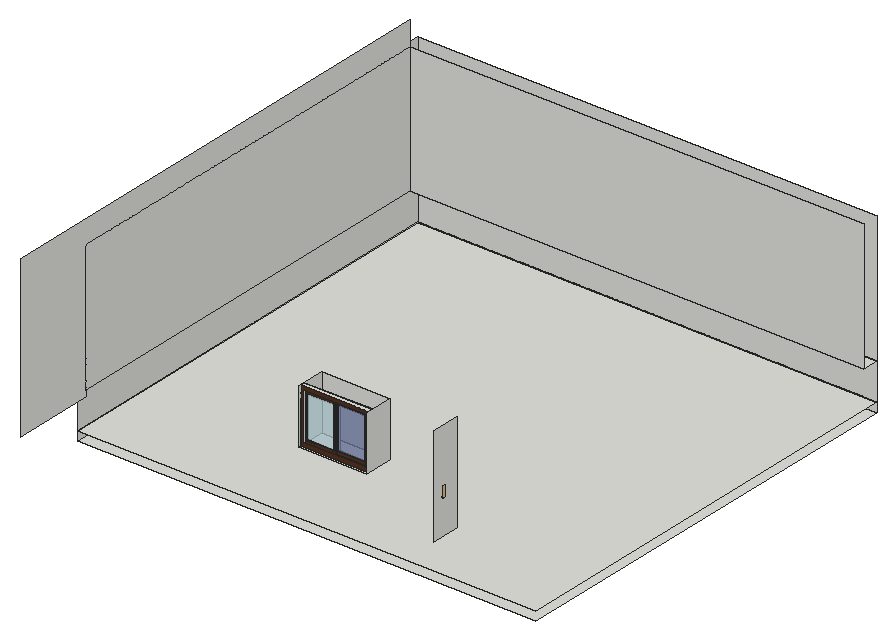
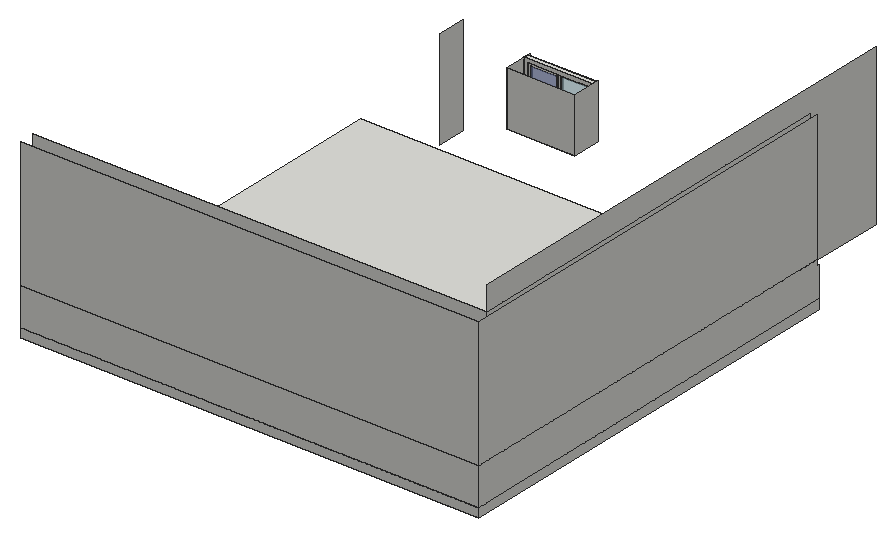
# SketchUp Ruby script. Lengths in inches.
U = 1.inch
M = Sketchup.active_model
def pt(a) = Geom::Point3d.new(a.map { |v| v * U })
def face(e, loops, mat)
  f = e.add_face(loops[0].map { |a| pt(a) })
  loops[1..].each { |l| e.add_face(l.map { |a| pt(a) }).erase! }
  f.material = f.back_material = mat if mat
  f
end
# faces: each face lists its corners as indices into pts; further lists are holes
def faces(e, pts, list, mat = nil) = list.each { |f| face(e, (f[0].is_a?(Array) ? f : [f]).map { |l| l.map { |i| pts[i] } }, mat) }
# xy, xz, yz: faces in a plane at the given z, y or x. An outline is a flat list of corners, or four numbers for a rectangle; further outlines are holes
def ring(l) = l.size == 4 ? [[l[0], l[1]], [l[2], l[1]], [l[2], l[3]], [l[0], l[3]]] : l.each_slice(2).to_a
def flat(e, list, mat, &to3) = list.each { |f| face(e, (f[0].is_a?(Array) ? f : [f]).map { |l| ring(l).map { |u, v| to3.(u, v) } }, mat) }
def xy(e, z, list, mat = nil) = flat(e, list, mat) { |x, y| [x, y, z] }
def xz(e, y, list, mat = nil) = flat(e, list, mat) { |x, z| [x, y, z] }
def yz(e, x, list, mat = nil) = flat(e, list, mat) { |y, z| [x, y, z] }
def lines(e, pts, list) = list.each { |a, b| e.add_line(pt(pts[a]), pt(pts[b])) }
# prism: a flat outline (further loops are holes) pulled along v
def prism(e, loops, v, mat = nil)
  f = face(e, loops, mat); d = Geom::Vector3d.new(v.map { |x| x * U })
  f.pushpull(f.normal.samedirection?(d) ? d.length : -d.length)
end
def box(e, o, s, mat = nil) = prism(e, [[o, [o[0] + s[0], o[1], o[2]], [o[0] + s[0], o[1] + s[1], o[2]], [o[0], o[1] + s[1], o[2]]]], [0, 0, s[2]], mat)
def at(x, y, z, deg = 0) = Geom::Transformation.translation(pt([x, y, z])) * Geom::Transformation.rotation(ORIGIN, Z_AXIS, deg.degrees)
def axes(o, x, y, z) = Geom::Transformation.new([*x, 0, *y, 0, *z, 0, *pt(o).to_a, 1])
def part(name) = M.definitions.add(name)
# library, detail: a bought-in or finely detailed component or shape, given as its bounding box
def library(name, o, s) = part(name).tap { |d| box(d.entities, o, s) }
def detail(e, o, s) = box(e.add_group.entities, o, s)
def put(e, d, t, mat = nil) = e.add_instance(d, t).tap { |i| i.material = mat if mat }
def group(e, t, mat = nil) = e.add_group.tap { |g| g.transformation = t; g.material = mat if mat }.entities
root = M.entities
M.materials.add("Material \#0").color = [86, 53, 35]
M.materials.add("Material \#1").color = [140, 140, 140]
M.materials.add("[Translucent_Glass_Safety]").color = [204, 235, 244]
M.materials["[Translucent_Glass_Safety]"].alpha = 0.5
M.materials.add("[Translucent_Glass_Sky_Reflection]").color = [125, 138, 183]
M.materials["[Translucent_Glass_Sky_Reflection]"].alpha = 0.52
c1 = part("Sliding window")
xy(c1.entities,0,[[0,0,4.33,55.51]])
xy(c1.entities,2.76,[[0,2.76,2,27.76],[3.15,2.76,4.33,27.76],[0,27.76,0.82,52.76],[0.82,27.76,2.36,52.76],[2.36,27.76,4.33,52.76]])
xy(c1.entities,4.72,[[2,4.72,2.4,26.38],[2.76,4.72,3.15,26.38],[0.82,29.13,1.22,50.79],[1.97,29.13,2.36,50.79]])
xy(c1.entities,36.61,[[2,4.72,2.4,26.38],[2.76,4.72,3.15,26.38],[0.82,29.13,1.22,50.79],[1.97,29.13,2.36,50.79]])
xy(c1.entities,38.58,[[0,2.76,2,27.76],[3.15,2.76,4.33,27.76],[0,27.76,0.82,52.76],[0.82,27.76,2.36,52.76],[2.36,27.76,4.33,52.76]])
xy(c1.entities,41.34,[[0,0,4.33,55.51]])
xz(c1.entities,0,[[0,0,4.33,41.34]])
xz(c1.entities,2.76,[[0,2.76,2,38.58],[3.15,2.76,4.33,38.58]])
xz(c1.entities,4.72,[[2,4.72,2.4,36.61],[2.76,4.72,3.15,36.61]])
xz(c1.entities,26.38,[[2,4.72,2.4,36.61],[2.76,4.72,3.15,36.61]])
xz(c1.entities,27.76,[[0.82,2.76,2,38.58],[2,2.76,2.36,38.58],[2.36,2.76,3.15,38.58]])
xz(c1.entities,29.13,[[0.82,4.72,1.22,36.61],[1.97,4.72,2.36,36.61]])
xz(c1.entities,50.79,[[0.82,4.72,1.22,36.61],[1.97,4.72,2.36,36.61]])
xz(c1.entities,52.76,[[0,2.76,0.82,38.58],[0.82,2.76,2.36,38.58],[2.36,2.76,4.33,38.58]])
xz(c1.entities,55.51,[[0,0,4.33,41.34]])
yz(c1.entities,0,[[[0,0,55.51,41.34],[2.76,2.76,52.76,38.58]]])
yz(c1.entities,0.82,[[[27.76,2.76,52.76,38.58],[29.13,4.72,50.79,36.61]]])
yz(c1.entities,1.22,[[29.13,4.72,50.79,36.61]],"[Translucent_Glass_Sky_Reflection]")
yz(c1.entities,1.97,[[29.13,4.72,50.79,36.61]],"[Translucent_Glass_Sky_Reflection]")
yz(c1.entities,2,[[[2.76,2.76,27.76,38.58],[4.72,4.72,26.38,36.61]]])
yz(c1.entities,2.36,[[[27.76,2.76,52.76,38.58],[29.13,4.72,50.79,36.61]]],"Material \#0")
yz(c1.entities,2.4,[[4.72,4.72,26.38,36.61]],"[Translucent_Glass_Safety]")
yz(c1.entities,2.76,[[4.72,4.72,26.38,36.61]],"[Translucent_Glass_Safety]")
yz(c1.entities,3.15,[[[2.76,2.76,27.76,38.58],[4.72,4.72,26.38,36.61]]],"Material \#0")
yz(c1.entities,4.33,[[[0,0,55.51,41.34],[2.76,2.76,52.76,38.58]]],"Material \#0")
c2 = library("3DGeom~4_Defintion",[-18.02,-499.97,-221.16],[36.04,1000,262.12])
c3 = part("3DGeom~5_Defintion")
xy(c3.entities,-225.24,[[-0.79,-499.98,-2.33,-499.64,7.45,-496.14],[-0.79,-499.98,7.45,-496.14,1.58,-499.88],[1.58,-499.88,7.45,-496.14,3.84,-499.16],[-2.33,-499.64,7.4,-485.75,7.45,-496.14],[3.84,-499.16,7.45,-496.14,5.85,-497.89],
  [7.45,-496.14,7.4,-485.75,8.24,-487.08],[7.45,-496.14,8.24,-487.08,8.96,-489.34],[7.45,-496.14,8.96,-489.34,9.0625,-491.71],[7.45,-496.14,9.0625,-491.71,8.55,-494.03],[-7.4,-496.08,-8.24,-494.76,2.32,-482.2],
  [-8.24,-494.76,-8.96,-492.5,2.32,-482.2],[-8.96,-492.5,-9.0625,-490.125,2.32,-482.2],[-9.0625,-490.125,-8.55,-487.81,2.32,-482.2],[-8.55,-487.81,-7.45,-485.7,2.32,-482.2],[-7.45,-485.7,-5.85,-483.95,2.32,-482.2],
  [-5.85,-483.95,-3.84,-482.68,2.32,-482.2],[-3.84,-482.68,-1.58,-481.96,2.32,-482.2],[2.32,-482.2,-1.58,-481.96,0.79,-481.86],[0,481.82,-2.35,482.13,-6.92,496.71],[0,481.82,-6.92,496.71,1.55,482.04],
  [-2.35,482.13,-4.55,483.04,-6.92,496.71],[-4.55,483.04,-6.43,484.49,-6.92,496.71],[-6.43,484.49,-7.88,486.37,-6.92,496.71],[6.92,485.12,-1.55,499.8125,7.88,495.47],[6.92,485.12,7.88,495.47,7.88,486.37],
  [-7.88,486.37,-8.79,488.57,-6.92,496.71],[7.88,486.37,7.88,495.47,8.79,488.57],[-8.79,488.57,-9.1,490.92,-6.92,496.71],[8.79,488.57,7.88,495.47,9.1,490.92],[-9.1,490.92,-8.79,493.28,-6.92,496.71],
  [9.1,490.92,7.88,495.47,8.79,493.28],[-8.79,493.28,-7.88,495.47,-6.92,496.71],[7.88,495.47,-1.55,499.8125,0,500.02],[7.88,495.47,0,500.02,2.35,499.71],[7.88,495.47,2.35,499.71,4.55,498.8],
  [7.88,495.47,4.55,498.8,6.43,497.35]],"Material \#1")
xy(c3.entities,-221.57,[[-2.33,-499.64,-5.22,-498.37,7.4,-485.75],[-5.22,-498.37,-7.4,-496.08,5.22,-483.47],[-5.22,-498.37,5.22,-483.47,7.4,-485.75],[-7.4,-496.08,2.32,-482.2,5.22,-483.47],[1.55,482.04,-6.92,496.71,-4.55,498.8],
  [1.55,482.04,-4.55,498.8,4.55,483.04],[4.55,483.04,-4.55,498.8,-1.55,499.8125],[4.55,483.04,-1.55,499.8125,6.92,485.12]],"Material \#1")
xy(c3.entities,38.05,[[-2.33,-499.64,7.4,-485.75,-5.22,-498.37],[-5.22,-498.37,5.22,-483.47,-7.4,-496.08],[-5.22,-498.37,7.4,-485.75,5.22,-483.47],[-7.4,-496.08,5.22,-483.47,2.32,-482.2],[1.55,482.04,-4.55,498.8,-6.92,496.71],
  [1.55,482.04,4.55,483.04,-4.55,498.8],[4.55,483.04,-1.55,499.8125,-4.55,498.8],[4.55,483.04,6.92,485.12,-1.55,499.8125]],"Material \#1")
xy(c3.entities,41.72,[[-0.79,-499.98,7.45,-496.14,-2.33,-499.64],[-0.79,-499.98,1.58,-499.88,7.45,-496.14],[1.58,-499.88,3.84,-499.16,7.45,-496.14],[-2.33,-499.64,7.45,-496.14,7.4,-485.75],[3.84,-499.16,5.85,-497.89,7.45,-496.14],
  [7.45,-496.14,8.24,-487.08,7.4,-485.75],[7.45,-496.14,8.55,-494.03,9.0625,-491.71],[7.45,-496.14,8.96,-489.34,8.24,-487.08],[7.45,-496.14,9.0625,-491.71,8.96,-489.34],[-7.4,-496.08,2.32,-482.2,-8.24,-494.76],
  [-8.24,-494.76,2.32,-482.2,-8.96,-492.5],[-8.96,-492.5,2.32,-482.2,-9.0625,-490.125],[-9.0625,-490.125,2.32,-482.2,-8.55,-487.81],[-8.55,-487.81,2.32,-482.2,-7.45,-485.7],[-7.45,-485.7,2.32,-482.2,-5.85,-483.95],
  [-5.85,-483.95,2.32,-482.2,-3.84,-482.68],[-3.84,-482.68,2.32,-482.2,-1.58,-481.96],[2.32,-482.2,0.79,-481.86,-1.58,-481.96],[0,481.82,-6.92,496.71,-2.35,482.13],[0,481.82,1.55,482.04,-6.92,496.71],
  [-2.35,482.13,-6.92,496.71,-4.55,483.04],[-4.55,483.04,-6.92,496.71,-6.43,484.49],[-6.43,484.49,-6.92,496.71,-7.88,486.37],[6.92,485.12,7.88,495.47,-1.55,499.8125],[6.92,485.12,7.88,486.37,7.88,495.47],
  [-7.88,486.37,-6.92,496.71,-8.79,488.57],[7.88,486.37,8.79,488.57,7.88,495.47],[-8.79,488.57,-6.92,496.71,-9.1,490.92],[8.79,488.57,9.1,490.92,7.88,495.47],[-9.1,490.92,-6.92,496.71,-8.79,493.28],
  [9.1,490.92,8.79,493.28,7.88,495.47],[-8.79,493.28,-6.92,496.71,-7.88,495.47],[7.88,495.47,0,500.02,-1.55,499.8125],[7.88,495.47,2.35,499.71,0,500.02],[7.88,495.47,4.55,498.8,2.35,499.71],
  [7.88,495.47,6.43,497.35,4.55,498.8]],"Material \#1")
xy(root,-42.8125,[[0,114.8125,424.88,508.6875]])
xy(root,-34.3125,[[0,114.8125,424.88,508.6875]])
xy(root,0,[[0,117.9375,4.88,117.9375,4.88,493.6875,424.88,493.6875,424.88,508.6875,0,508.6875]])
xy(root,24.47,[[205.2,114.8125,268.45,141.3125]])
xz(root,116.5625,[[337.22,27.35,337.09,27.37,337.22,27.37],[337.09,27.37,336.97,27.4,337.09,27.38],[337.09,27.37,337.09,27.38,337.22,27.37],[337.09,27.38,336.97,27.4,336.97,27.41],[336.97,27.4,336.85,27.46,336.97,27.41],
  [336.97,27.41,336.85,27.46,336.86,27.47],[336.86,27.47,336.75,27.53,336.76,27.54],[336.75,27.53,336.67,27.62,336.76,27.54],[336.76,27.54,336.67,27.62,336.68,27.63],[337.14,27.57,337.1,27.59,337.14,27.58],
  [337.14,27.58,337.1,27.59,337.1,27.6],[337.1,27.59,337.0625,27.61,337.1,27.6],[337.1,27.6,337.0625,27.61,337.07,27.625],[337.0625,27.61,337.04,27.64,337.07,27.625],[336.67,27.62,336.6,27.72,336.68,27.63],
  [337.07,27.625,337.04,27.64,337.04,27.65],[336.68,27.63,336.6,27.72,336.61,27.73],[337.04,27.64,337.01,27.68,337.04,27.65],[337.04,27.65,337.01,27.68,337.02,27.69],[337.01,27.68,336.99,27.72,337.02,27.69],
  [337.02,27.69,336.99,27.72,337.01,27.72],[336.6,27.72,336.54,27.84,336.61,27.73],[336.99,27.72,336.98,27.76,337.01,27.72],[337.01,27.72,336.98,27.76,336.99,27.76],[336.61,27.73,336.54,27.84,336.55,27.85],
  [336.98,27.76,336.98,27.8,336.99,27.76],[336.99,27.76,336.98,27.8,336.99,27.8],[336.98,27.8,336.98,27.85,336.99,27.8],[336.99,27.8,336.98,27.85,336.99,27.85],[336.54,27.84,336.51,27.97,336.55,27.85],
  [336.55,27.85,336.51,27.97,336.52,27.97],[336.98,27.85,336.99,27.89,336.99,27.85],[336.99,27.85,336.99,27.89,337.01,27.89],[336.99,27.89,337.01,27.93,337.01,27.89],[337.01,27.89,337.01,27.93,337.02,27.92],
  [337.02,27.92,337.01,27.93,337.04,27.97],[337.02,27.92,337.04,27.97,337.04,27.96],[337.04,27.96,337.04,27.97,337.0625,28],[337.04,27.96,337.0625,28,337.07,27.99],[336.51,27.97,336.5,28.11,336.52,27.97],
  [336.52,27.97,336.5,28.11,336.51,28.11],[337.07,27.99,337.0625,28,337.1,28.02],[337.07,27.99,337.1,28.02,337.1,28.01],[337.1,28.01,337.1,28.02,337.14,28.04],[337.1,28.01,337.14,28.04,337.14,28.03],
  [337.14,28.03,337.14,28.04,337.18,28.05],[337.14,28.03,337.18,28.05,337.18,28.04],[337.18,28.04,337.18,28.05,337.22,28.05],[337.18,28.04,337.22,28.05,337.22,28.04]],"Material \#1")
xz(root,117.9375,[[0,-5.75,4.88,0]])
xz(root,118.74,[[337.22,27.35,337.22,27.37,337.09,27.37],[337.09,27.37,337.09,27.38,336.97,27.4],[337.09,27.37,337.22,27.37,337.09,27.38],[337.09,27.38,336.97,27.41,336.97,27.4],[336.97,27.4,336.97,27.41,336.85,27.46],
  [336.97,27.41,336.86,27.47,336.85,27.46],[336.85,27.46,336.86,27.47,336.75,27.53],[336.86,27.47,336.76,27.54,336.75,27.53],[336.75,27.53,336.76,27.54,336.67,27.62],[336.76,27.54,336.68,27.63,336.67,27.62],
  [337.18,27.56,337.18,27.57,337.14,27.57],[337.18,27.56,337.22,27.56,337.22,27.57],[337.18,27.56,337.22,27.57,337.18,27.57],[337.14,27.57,337.14,27.58,337.1,27.59],[337.14,27.57,337.18,27.57,337.14,27.58],
  [337.14,27.58,337.1,27.6,337.1,27.59],[337.1,27.59,337.1,27.6,337.0625,27.61],[337.1,27.6,337.07,27.625,337.0625,27.61],[337.0625,27.61,337.07,27.625,337.04,27.64],[336.67,27.62,336.68,27.63,336.6,27.72],
  [337.07,27.625,337.04,27.65,337.04,27.64],[336.68,27.63,336.61,27.73,336.6,27.72],[337.04,27.64,337.04,27.65,337.01,27.68],[337.04,27.65,337.02,27.69,337.01,27.68],[337.01,27.68,337.02,27.69,336.99,27.72],
  [337.02,27.69,337.01,27.72,336.99,27.72],[336.6,27.72,336.61,27.73,336.54,27.84],[336.99,27.72,337.01,27.72,336.98,27.76],[337.01,27.72,336.99,27.76,336.98,27.76],[336.61,27.73,336.55,27.85,336.54,27.84],
  [336.98,27.76,336.99,27.76,336.98,27.8],[336.99,27.76,336.99,27.8,336.98,27.8],[336.98,27.8,336.99,27.8,336.98,27.85],[336.99,27.8,336.99,27.85,336.98,27.85],[336.54,27.84,336.55,27.85,336.51,27.97],
  [336.55,27.85,336.52,27.97,336.51,27.97],[336.98,27.85,336.99,27.85,336.99,27.89],[336.99,27.85,337.01,27.89,336.99,27.89],[336.99,27.89,337.01,27.89,337.01,27.93],[337.01,27.89,337.02,27.92,337.01,27.93],
  [337.02,27.92,337.04,27.97,337.01,27.93],[337.02,27.92,337.04,27.96,337.04,27.97],[337.04,27.96,337.0625,28,337.04,27.97],[337.04,27.96,337.07,27.99,337.0625,28],[336.51,27.97,336.52,27.97,336.5,28.11],
  [336.52,27.97,336.51,28.11,336.5,28.11],[337.07,27.99,337.1,28.02,337.0625,28],[337.07,27.99,337.1,28.01,337.1,28.02],[337.1,28.01,337.14,28.03,337.14,28.04],[337.1,28.01,337.14,28.04,337.1,28.02],
  [337.14,28.03,337.18,28.04,337.18,28.05],[337.14,28.03,337.18,28.05,337.14,28.04],[337.18,28.04,337.22,28.04,337.22,28.05],[337.18,28.04,337.22,28.05,337.18,28.05],[336.5,28.11,336.51,28.11,336.5,36.6875],
  [336.51,28.11,336.51,36.6875,336.5,36.6875]],"Material \#1")
xz(root,141.3125,[[205.2,24.47,268.45,75.1]])
xz(root,493.6875,[[4.88,0,424.88,120]])
xz(root,508.6875,[[0,-42.8125,424.88,-34.3125],[0,-34.3125,424.88,0],[0,0,424.88,120]])
yz(root,0,[[114.8125,-42.8125,508.6875,-34.3125],[114.8125,-34.3125,114.8125,-5.75,117.9375,-5.75,117.9375,0,508.6875,0,508.6875,-34.3125],[117.9375,0,508.6875,120]])
yz(root,4.88,[[42.5,-5.75,117.9375,-5.75,117.9375,120,493.6875,120,493.6875,141.9375,42.5,141.9375],[117.9375,0,493.6875,120]])
yz(root,205.2,[[114.8125,24.47,141.3125,75.1]])
yz(root,268.45,[[114.8125,24.47,141.3125,75.1]])
yz(root,330.35,[[114.8125,-10.53,141.3125,81.34]])
p = [[337.15,116.56,27.76],[337.15,116.59,27.76],[337.14,116.59,27.73],[337.14,116.5625,27.73],[337.12,116.6,27.71],[337.12,116.57,27.71],
  [337.14,116.6,27.6875],[337.14,116.57,27.6875],[337.16,116.6,27.67],[337.16,116.57,27.67],[337.18,116.59,27.7],[337.18,116.5625,27.7],
  [337.2,116.59,27.72],[337.2,116.56,27.72],[337.29,116.59,27.85],[337.29,116.56,27.85],[337.24,116.56,27.89],[337.24,116.59,27.89],
  [337.26,116.5625,27.91],[337.26,116.59,27.91],[337.3,116.59,27.88],[337.3,116.5625,27.88],[337.32,116.6,27.9],[337.32,116.57,27.9],
  [337.3,116.6,27.92],[337.3,116.57,27.92],[337.27,116.6,27.9375],[337.27,116.57,27.9375]]
faces(root,p,[[0,1,2],[2,3,0],[3,2,4],[4,5,3],[5,4,6],[6,7,5],[7,6,8],[8,9,7],
  [9,8,10],[10,11,9],[11,10,12],[12,13,11],[13,12,14],[14,15,13],[16,17,1],[1,0,16],
  [18,19,17],[17,16,18],[15,14,20],[20,21,15],[21,20,22],[22,23,21],[23,22,24],[24,25,23],
  [25,24,26],[26,27,25],[27,26,19],[19,18,27]],"Material \#1")
put(root,c1,axes([205.2,120.8125,24.47],[0,-1,0],[1.1394,0,0],[0,0,1.22464]))
put(root,c2,axes([337.22,118.4,32.4],[0.00916,0,0],[0,0,0.00953],[0,0.00833,0]),"Material \#1")
put(root,c3,axes([337.22,118.4,32.4],[0.00899,0,0],[0,0,0.00936],[0,0.00818,0]),"Material \#1")
